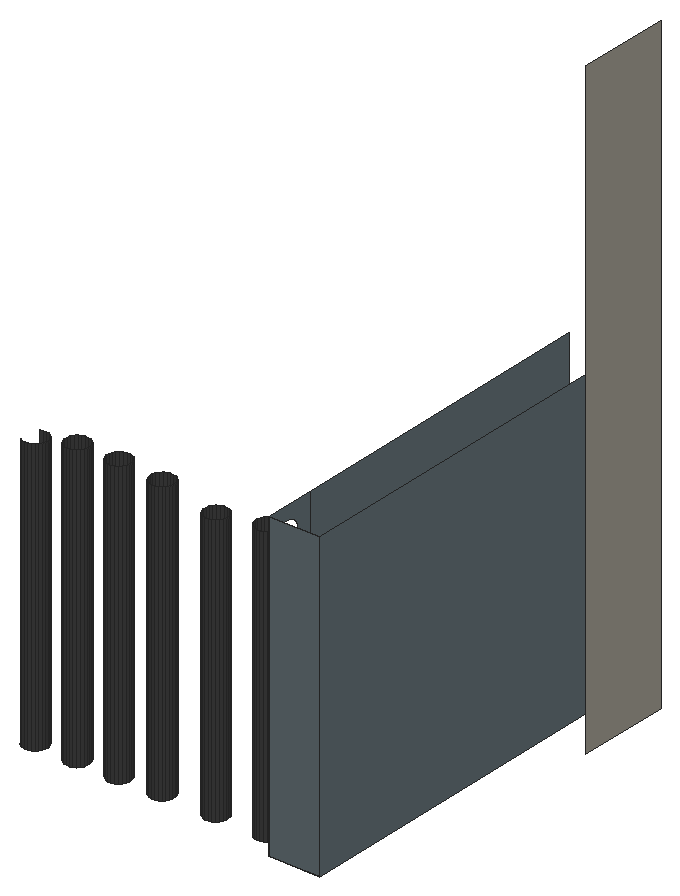
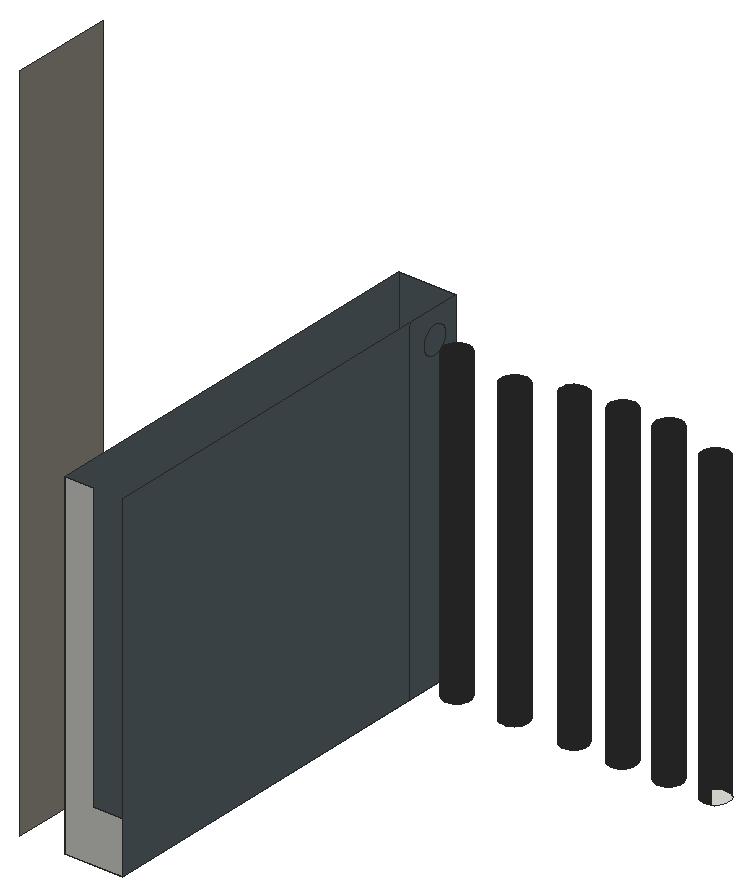
# SketchUp Ruby script. Lengths in inches.
U = 1.inch
M = Sketchup.active_model
def pt(a) = Geom::Point3d.new(a.map { |v| v * U })
def face(e, loops, mat)
  f = e.add_face(loops[0].map { |a| pt(a) })
  loops[1..].each { |l| e.add_face(l.map { |a| pt(a) }).erase! }
  f.material = f.back_material = mat if mat
  f
end
# faces: each face lists its corners as indices into pts; further lists are holes
def faces(e, pts, list, mat = nil) = list.each { |f| face(e, (f[0].is_a?(Array) ? f : [f]).map { |l| l.map { |i| pts[i] } }, mat) }
# xy, xz, yz: faces in a plane at the given z, y or x. An outline is a flat list of corners, or four numbers for a rectangle; further outlines are holes
def ring(l) = l.size == 4 ? [[l[0], l[1]], [l[2], l[1]], [l[2], l[3]], [l[0], l[3]]] : l.each_slice(2).to_a
def flat(e, list, mat, &to3) = list.each { |f| face(e, (f[0].is_a?(Array) ? f : [f]).map { |l| ring(l).map { |u, v| to3.(u, v) } }, mat) }
def xy(e, z, list, mat = nil) = flat(e, list, mat) { |x, y| [x, y, z] }
def xz(e, y, list, mat = nil) = flat(e, list, mat) { |x, z| [x, y, z] }
def yz(e, x, list, mat = nil) = flat(e, list, mat) { |y, z| [x, y, z] }
def lines(e, pts, list) = list.each { |a, b| e.add_line(pt(pts[a]), pt(pts[b])) }
# prism: a flat outline (further loops are holes) pulled along v
def prism(e, loops, v, mat = nil)
  f = face(e, loops, mat); d = Geom::Vector3d.new(v.map { |x| x * U })
  f.pushpull(f.normal.samedirection?(d) ? d.length : -d.length)
end
def box(e, o, s, mat = nil) = prism(e, [[o, [o[0] + s[0], o[1], o[2]], [o[0] + s[0], o[1] + s[1], o[2]], [o[0], o[1] + s[1], o[2]]]], [0, 0, s[2]], mat)
def at(x, y, z, deg = 0) = Geom::Transformation.translation(pt([x, y, z])) * Geom::Transformation.rotation(ORIGIN, Z_AXIS, deg.degrees)
def axes(o, x, y, z) = Geom::Transformation.new([*x, 0, *y, 0, *z, 0, *pt(o).to_a, 1])
def part(name) = M.definitions.add(name)
# library, detail: a bought-in or finely detailed component or shape, given as its bounding box
def library(name, o, s) = part(name).tap { |d| box(d.entities, o, s) }
def detail(e, o, s) = box(e.add_group.entities, o, s)
def put(e, d, t, mat = nil) = e.add_instance(d, t).tap { |i| i.material = mat if mat }
def group(e, t, mat = nil) = e.add_group.tap { |g| g.transformation = t; g.material = mat if mat }.entities
root = M.entities
M.materials.add("[Color M07]").color = [58, 58, 58]
M.materials.add("[Formica Graystone]").color = [149, 146, 135]
M.materials.add("[Formica Speckled Grey]").color = [94, 105, 111]
xy(root,452.9,[[292.38,118.22,295.93,144.04],[274.78,119.22,274.57,119.27,274.39,119.375,274.23,119.52,274.125,119.71,274.07,119.91,274.07,120.125,274.12,120.33,274.22,120.51,274.37,120.67,274.55,120.77,274.76,120.83,274.97,120.83,275.18,120.78,275.36,120.68,275.51,120.53,275.62,120.35,275.68,120.14,275.68,119.93,275.63,119.72,275.52,119.54,275.375,119.39,275.19,119.28,274.99,119.22],[277.65,119.22,277.45,119.27,277.26,119.375,277.11,119.52,277,119.71,276.94,119.91,276.94,120.125,277,120.33,277.1,120.51,277.25,120.67,277.43,120.77,277.63,120.83,277.85,120.83,278.05,120.78,278.24,120.68,278.39,120.53,278.5,120.35,278.55,120.14,278.56,119.93,278.5,119.72,278.4,119.54,278.25,119.39,278.07,119.28,277.86,119.22],[280.53,119.22,280.32,119.27,280.14,119.375,279.98,119.52,279.875,119.71,279.82,119.91,279.82,120.125,279.87,120.33,279.97,120.51,280.12,120.67,280.3,120.77,280.51,120.83,280.72,120.83,280.93,120.78,281.11,120.68,281.26,120.53,281.37,120.35,281.43,120.14,281.43,119.93,281.38,119.72,281.27,119.54,281.125,119.39,280.94,119.28,280.74,119.22],[283.53,119.22,283.32,119.27,283.14,119.375,282.98,119.52,282.875,119.71,282.82,119.91,282.82,120.125,282.87,120.33,282.97,120.51,283.12,120.67,283.3,120.77,283.51,120.83,283.72,120.83,283.93,120.78,284.11,120.68,284.26,120.53,284.37,120.35,284.43,120.14,284.43,119.93,284.38,119.72,284.27,119.54,284.125,119.39,283.94,119.28,283.74,119.22],
  [287.21,119.22,287.01,119.27,286.82,119.375,286.67,119.52,286.5625,119.71,286.51,119.91,286.5,120.125,286.56,120.33,286.66,120.51,286.81,120.67,286.99,120.77,287.2,120.83,287.41,120.83,287.61,120.78,287.8,120.68,287.95,120.53,288.06,120.35,288.12,120.14,288.12,119.93,288.07,119.72,287.96,119.54,287.8125,119.39,287.63,119.28,287.43,119.22],[290.78,119.22,290.57,119.27,290.39,119.375,290.23,119.52,290.125,119.71,290.07,119.91,290.07,120.125,290.12,120.33,290.22,120.51,290.37,120.67,290.55,120.77,290.76,120.83,290.97,120.83,291.18,120.78,291.36,120.68,291.51,120.53,291.62,120.35,291.68,120.14,291.68,119.93,291.63,119.72,291.52,119.54,291.375,119.39,291.19,119.28,290.99,119.22]])
xz(root,118.22,[[292.38,452.9,295.93,473.83]],"[Formica Speckled Grey]")
xz(root,119.22,[[274.78,452.9,274.99,471.83],[277.65,452.9,277.86,472.48],[280.53,452.9,280.74,472.48],[283.53,452.9,283.74,472.27],[287.21,452.9,287.43,471.52],
  [290.78,452.9,290.99,472.05]],"[Color M07]")
xz(root,120.83,[[274.76,452.9,274.97,471.83],[277.63,452.9,277.85,472.48],[280.51,452.9,280.72,472.48],[283.51,452.9,283.72,472.27],[287.2,452.9,287.41,471.52],
  [290.76,452.9,290.97,472.05]],"[Color M07]")
xz(root,144.04,[[292.38,452.9,295.93,452.9,295.93,473.83,294.2,473.83,294.2,456.09,292.38,456.09]])
yz(root,275.68,[[119.93,452.9,120.14,471.83]],"[Color M07]")
yz(root,276.94,[[119.91,452.9,120.125,472.48]],"[Color M07]")
yz(root,279.82,[[119.91,452.9,120.125,472.48]],"[Color M07]")
yz(root,281.43,[[119.93,452.9,120.14,472.48]],"[Color M07]")
yz(root,282.82,[[119.91,452.9,120.125,472.27]],"[Color M07]")
yz(root,284.43,[[119.93,452.9,120.14,472.27]],"[Color M07]")
yz(root,288.12,[[119.93,452.9,120.14,471.52]],"[Color M07]")
yz(root,290.07,[[119.91,452.9,120.125,472.05]],"[Color M07]")
yz(root,291.68,[[119.93,452.9,120.14,472.05]],"[Color M07]")
yz(root,292.38,[[[118.22,452.9,121.78,473.83],[119.86,471.17,120.09,471.2,120.3,471.29,120.48,471.43,120.62,471.61,120.71,471.82,120.74,472.05,120.71,472.27,120.62,472.48,120.48,472.67,120.3,472.81,120.09,472.89,119.86,472.92,119.64,472.89,119.42,472.81,119.24,472.67,119.1,472.48,119.02,472.27,118.99,472.05,119.02,471.82,119.1,471.61,119.24,471.43,119.42,471.29,119.64,471.2]],[121.78,452.9,144.04,473.83]],"[Formica Speckled Grey]")
yz(root,295.93,[[118.22,452.9,144.04,473.83]],"[Formica Speckled Grey]")
yz(root,298.71,[[137.66,452.9,144.04,495.36]],"[Formica Graystone]")
p = [[274.57,119.27,452.9],[274.78,119.22,452.9],[274.78,119.22,471.83],[274.57,119.27,471.83],[274.99,119.22,452.9],[275.19,119.28,452.9],
  [275.19,119.28,471.83],[274.99,119.22,471.83],[277.45,119.27,452.9],[277.65,119.22,452.9],[277.65,119.22,472.48],[277.45,119.27,472.48],
  [277.86,119.22,452.9],[278.07,119.28,452.9],[278.07,119.28,472.48],[277.86,119.22,472.48],[280.32,119.27,452.9],[280.53,119.22,452.9],
  [280.53,119.22,472.48],[280.32,119.27,472.48],[280.74,119.22,452.9],[280.94,119.28,452.9],[280.94,119.28,472.48],[280.74,119.22,472.48],
  [283.32,119.27,452.9],[283.53,119.22,452.9],[283.53,119.22,472.27],[283.32,119.27,472.27],[283.74,119.22,452.9],[283.94,119.28,452.9],
  [283.94,119.28,472.27],[283.74,119.22,472.27],[287.01,119.27,452.9],[287.21,119.22,452.9],[287.21,119.22,471.52],[287.01,119.27,471.52],
  [287.43,119.22,452.9],[287.63,119.28,452.9],[287.63,119.28,471.52],[287.43,119.22,471.52],[290.57,119.27,452.9],[290.78,119.22,452.9],
  [290.78,119.22,472.05],[290.57,119.27,472.05],[290.99,119.22,452.9],[291.19,119.28,452.9],[291.19,119.28,472.05],[290.99,119.22,472.05],
  [274.39,119.375,452.9],[274.39,119.375,471.83],[275.375,119.39,452.9],[275.375,119.39,471.83],[277.26,119.375,452.9],[277.26,119.375,472.48],
  [278.25,119.39,452.9],[278.25,119.39,472.48],[280.14,119.375,452.9],[280.14,119.375,472.48],[281.125,119.39,452.9],[281.125,119.39,472.48],
  [283.14,119.375,452.9],[283.14,119.375,472.27],[284.125,119.39,452.9],[284.125,119.39,472.27],[286.82,119.375,452.9],[286.82,119.375,471.52],
  [287.8125,119.39,452.9],[287.8125,119.39,471.52],[290.39,119.375,452.9],[290.39,119.375,472.05],[291.375,119.39,452.9],[291.375,119.39,472.05],
  [275.52,119.54,452.9],[275.52,119.54,471.83],[277.11,119.52,452.9],[277.11,119.52,472.48],[278.4,119.54,452.9],[278.4,119.54,472.48],
  [279.98,119.52,452.9],[279.98,119.52,472.48],[281.27,119.54,452.9],[281.27,119.54,472.48],[282.98,119.52,452.9],[282.98,119.52,472.27],
  [284.27,119.54,452.9],[284.27,119.54,472.27],[286.67,119.52,452.9],[286.67,119.52,471.52],[287.96,119.54,452.9],[287.96,119.54,471.52],
  [290.23,119.52,452.9],[290.23,119.52,472.05],[291.52,119.54,452.9],[291.52,119.54,472.05],[275.63,119.72,452.9],[275.63,119.72,471.83],
  [277,119.71,452.9],[277,119.71,472.48],[278.5,119.72,452.9],[278.5,119.72,472.48],[279.875,119.71,452.9],[279.875,119.71,472.48],
  [281.38,119.72,452.9],[281.38,119.72,472.48],[282.875,119.71,452.9],[282.875,119.71,472.27],[284.38,119.72,452.9],[284.38,119.72,472.27],
  [286.5625,119.71,452.9],[286.5625,119.71,471.52],[288.07,119.72,452.9],[288.07,119.72,471.52],[290.125,119.71,452.9],[290.125,119.71,472.05],
  [291.63,119.72,452.9],[291.63,119.72,472.05],[275.68,119.93,452.9],[275.68,119.93,471.83],[276.94,119.91,452.9],[276.94,119.91,472.48],
  [278.56,119.93,452.9],[278.56,119.93,472.48],[279.82,119.91,452.9],[279.82,119.91,472.48],[281.43,119.93,452.9],[281.43,119.93,472.48],
  [282.82,119.91,452.9],[282.82,119.91,472.27],[284.43,119.93,452.9],[284.43,119.93,472.27],[286.51,119.91,452.9],[286.51,119.91,471.52],
  [288.12,119.93,452.9],[288.12,119.93,471.52],[290.07,119.91,452.9],[290.07,119.91,472.05],[291.68,119.93,452.9],[291.68,119.93,472.05],
  [278.55,120.14,452.9],[278.55,120.14,472.48],[286.5,120.125,452.9],[286.5,120.125,471.52],[275.68,120.14,452.9],[275.62,120.35,452.9],
  [275.62,120.35,471.83],[275.68,120.14,471.83],[277,120.33,452.9],[276.94,120.125,452.9],[276.94,120.125,472.48],[277,120.33,472.48],
  [278.5,120.35,452.9],[278.5,120.35,472.48],[279.87,120.33,452.9],[279.82,120.125,452.9],[279.82,120.125,472.48],[279.87,120.33,472.48],
  [281.43,120.14,452.9],[281.37,120.35,452.9],[281.37,120.35,472.48],[281.43,120.14,472.48],[282.87,120.33,452.9],[282.82,120.125,452.9],
  [282.82,120.125,472.27],[282.87,120.33,472.27],[284.43,120.14,452.9],[284.37,120.35,452.9],[284.37,120.35,472.27],[284.43,120.14,472.27],
  [286.56,120.33,452.9],[286.56,120.33,471.52],[288.12,120.14,452.9],[288.06,120.35,452.9],[288.06,120.35,471.52],[288.12,120.14,471.52],
  [290.12,120.33,452.9],[290.07,120.125,452.9],[290.07,120.125,472.05],[290.12,120.33,472.05],[291.68,120.14,452.9],[291.62,120.35,452.9],
  [291.62,120.35,472.05],[291.68,120.14,472.05],[275.51,120.53,452.9],[275.51,120.53,471.83],[277.1,120.51,452.9],[277.1,120.51,472.48],
  [278.39,120.53,452.9],[278.39,120.53,472.48],[279.97,120.51,452.9],[279.97,120.51,472.48],[281.26,120.53,452.9],[281.26,120.53,472.48],
  [282.97,120.51,452.9],[282.97,120.51,472.27],[284.26,120.53,452.9],[284.26,120.53,472.27],[286.66,120.51,452.9],[286.66,120.51,471.52],
  [287.95,120.53,452.9],[287.95,120.53,471.52],[290.22,120.51,452.9],[290.22,120.51,472.05],[291.51,120.53,452.9],[291.51,120.53,472.05],
  [275.36,120.68,452.9],[275.36,120.68,471.83],[277.25,120.67,452.9],[277.2,120.62,472.48],[277.25,120.67,472.48],[278.24,120.68,452.9],
  [278.24,120.68,472.48],[278.29,120.62,472.48],[280.12,120.67,452.9],[280.08,120.62,472.48],[280.12,120.67,472.48],[281.11,120.68,452.9],
  [281.11,120.68,472.48],[281.17,120.62,472.48],[283.12,120.67,452.9],[283.12,120.67,472.27],[284.11,120.68,452.9],[284.11,120.68,472.27],
  [286.81,120.67,452.9],[286.81,120.67,471.52],[287.8,120.68,452.9],[287.8,120.68,471.52],[290.37,120.67,452.9],[290.37,120.67,472.05],
  [291.36,120.68,452.9],[291.36,120.68,472.05],[275.18,120.78,452.9],[275.18,120.78,471.83],[277.43,120.77,452.9],[277.43,120.77,472.48],
  [278.05,120.78,452.9],[278.05,120.78,472.48],[280.3,120.77,452.9],[280.3,120.77,472.48],[280.93,120.78,452.9],[280.93,120.78,472.48],
  [283.3,120.77,452.9],[283.19,120.71,472.27],[283.3,120.77,472.27],[283.93,120.78,452.9],[283.93,120.78,472.27],[284.06,120.71,472.27],
  [286.99,120.77,452.9],[286.99,120.77,471.52],[287.61,120.78,452.9],[287.61,120.78,471.52],[290.55,120.77,452.9],[290.49,120.74,472.05],
  [290.55,120.77,472.05],[291.18,120.78,452.9],[291.18,120.78,472.05],[291.25,120.74,472.05],[274.76,120.83,452.9],[274.55,120.77,452.9],
  [274.55,120.77,471.83],[274.76,120.83,471.83],[274.97,120.83,452.9],[274.97,120.83,471.83],[277.63,120.83,452.9],[277.63,120.83,472.48],
  [277.85,120.83,452.9],[277.85,120.83,472.48],[280.51,120.83,452.9],[280.51,120.83,472.48],[280.72,120.83,452.9],[280.72,120.83,472.48],
  [283.51,120.83,452.9],[283.51,120.83,472.27],[283.72,120.83,452.9],[283.72,120.83,472.27],[287.2,120.83,452.9],[287.2,120.83,471.52],
  [287.41,120.83,452.9],[287.41,120.83,471.52],[290.76,120.83,452.9],[290.76,120.83,472.05],[290.97,120.83,452.9],[290.97,120.83,472.05]]
faces(root,p,[[0,1,2,3],[4,5,6,7],[8,9,10,11],[12,13,14,15],[16,17,18,19],[20,21,22,23],[24,25,26,27],[28,29,30,31],
  [32,33,34,35],[36,37,38,39],[40,41,42,43],[44,45,46,47],[48,0,3,49],[5,50,51,6],[52,8,11,53],[13,54,55,14],
  [56,16,19,57],[21,58,59,22],[60,24,27,61],[29,62,63,30],[64,32,35,65],[37,66,67,38],[68,40,43,69],[45,70,71,46],
  [50,72,73,51],[74,52,53,75],[54,76,77,55],[78,56,57,79],[58,80,81,59],[82,60,61,83],[62,84,85,63],[86,64,65,87],
  [66,88,89,67],[90,68,69,91],[70,92,93,71],[72,94,95,73],[96,74,75,97],[76,98,99,77],[100,78,79,101],[80,102,103,81],
  [104,82,83,105],[84,106,107,85],[108,86,87,109],[88,110,111,89],[112,90,91,113],[92,114,115,93],[94,116,117,95],[118,96,97,119],
  [98,120,121,99],[122,100,101,123],[102,124,125,103],[126,104,105,127],[106,128,129,107],[130,108,109,131],[110,132,133,111],[134,112,113,135],
  [114,136,137,115],[120,138,139,121],[140,130,131,141],[142,143,144,145],[146,147,148,149],[138,150,151,139],[152,153,154,155],[156,157,158,159],
  [160,161,162,163],[164,165,166,167],[168,140,141,169],[170,171,172,173],[174,175,176,177],[178,179,180,181],[143,182,183,144],[184,146,149,185],
  [150,186,187,151],[188,152,155,189],[157,190,191,158],[192,160,163,193],[165,194,195,166],[196,168,169,197],[171,198,199,172],[200,174,177,201],
  [179,202,203,180],[182,204,205,183],[206,184,185,207,208],[186,209,210,211,187],[212,188,189,213,214],[190,215,216,217,191],[218,192,193,219],[194,220,221,195],
  [222,196,197,223],[198,224,225,199],[226,200,201,227],[202,228,229,203],[204,230,231,205],[232,206,208,233],[209,234,235,210],[236,212,214,237],
  [215,238,239,216],[240,218,219,241,242],[220,243,244,245,221],[246,222,223,247],[224,248,249,225],[250,226,227,251,252],[228,253,254,255,229],[256,257,258,259],
  [230,260,261,231],[262,232,233,263],[234,264,265,235],[266,236,237,267],[238,268,269,239],[270,240,242,271],[243,272,273,244],[274,246,247,275],
  [248,276,277,249],[278,250,252,279],[253,280,281,254]],"[Color M07]")
